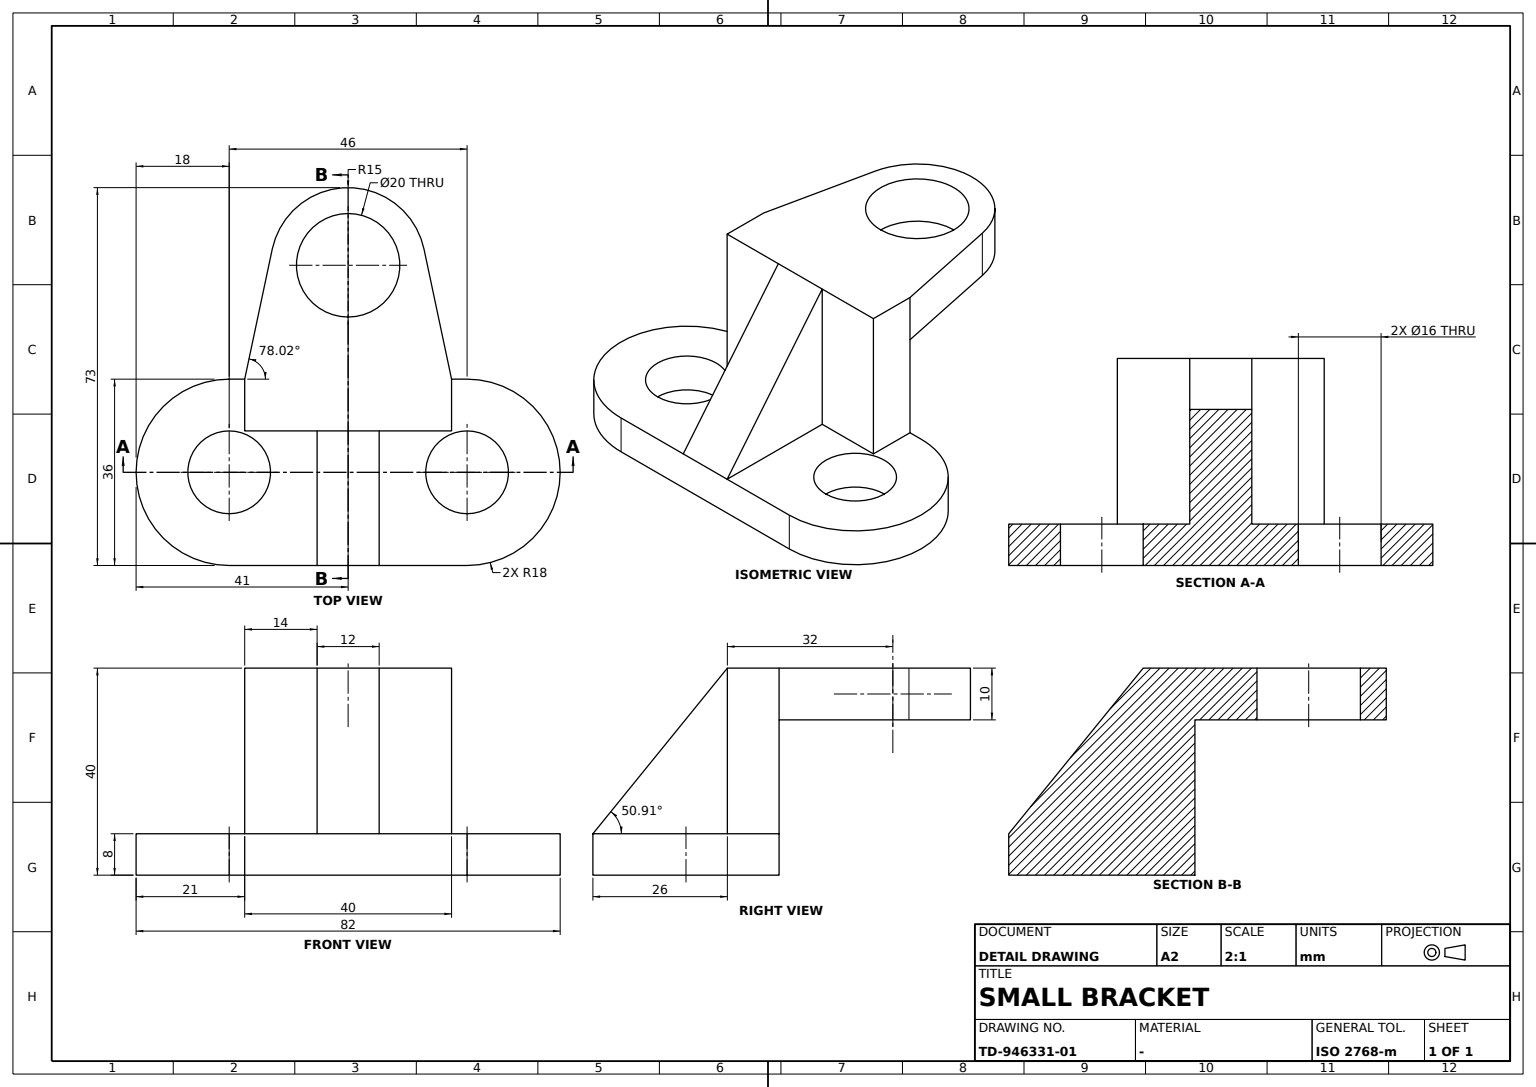
ISO-10303-21;
HEADER;
FILE_DESCRIPTION((''),'2;1');
FILE_NAME('','',(''),(''),'','','');
FILE_SCHEMA(('AUTOMOTIVE_DESIGN'));
ENDSEC;
DATA;
#1=APPLICATION_CONTEXT('');
#2=PRODUCT_CONTEXT('',#1,'mechanical');
#3=PRODUCT('','','',(#2));
#4=PRODUCT_DEFINITION_FORMATION('','',#3);
#5=PRODUCT_DEFINITION_CONTEXT('',#1,'design');
#6=PRODUCT_DEFINITION('','',#4,#5);
#7=PRODUCT_DEFINITION_SHAPE('','',#6);
#8=(LENGTH_UNIT()NAMED_UNIT(*)SI_UNIT(.MILLI.,.METRE.));
#9=(NAMED_UNIT(*)PLANE_ANGLE_UNIT()SI_UNIT($,.RADIAN.));
#10=(NAMED_UNIT(*)SI_UNIT($,.STERADIAN.)SOLID_ANGLE_UNIT());
#11=UNCERTAINTY_MEASURE_WITH_UNIT(LENGTH_MEASURE(0.005),#8,'distance_accuracy_value','');
#12=(GEOMETRIC_REPRESENTATION_CONTEXT(3)GLOBAL_UNCERTAINTY_ASSIGNED_CONTEXT((#11))GLOBAL_UNIT_ASSIGNED_CONTEXT((#8,#9,#10))REPRESENTATION_CONTEXT('',''));
#13=CARTESIAN_POINT('',(-30.,0.,26.));
#14=VERTEX_POINT('',#13);
#15=CARTESIAN_POINT('',(-40.,0.,26.));
#16=DIRECTION('',(0.,0.,1.));
#17=DIRECTION('',(1.,0.,0.));
#18=AXIS2_PLACEMENT_3D('',#15,#16,#17);
#19=CIRCLE('',#18,10.);
#20=EDGE_CURVE('',#14,#14,#19,.T.);
#21=ORIENTED_EDGE('',*,*,#20,.F.);
#22=EDGE_LOOP('',(#21));
#23=FACE_BOUND('',#22,.T.);
#24=CARTESIAN_POINT('',(-30.,0.,36.));
#25=VERTEX_POINT('',#24);
#26=CARTESIAN_POINT('',(-40.,0.,36.));
#27=AXIS2_PLACEMENT_3D('',#26,#16,#17);
#28=CIRCLE('',#27,10.);
#29=EDGE_CURVE('',#25,#25,#28,.T.);
#30=ORIENTED_EDGE('',*,*,#29,.T.);
#31=EDGE_LOOP('',(#30));
#32=FACE_BOUND('',#31,.T.);
#33=CARTESIAN_POINT('',(-40.,0.,31.));
#34=DIRECTION('',(0.,1.,0.));
#35=AXIS2_PLACEMENT_3D('',#33,#16,#34);
#36=CYLINDRICAL_SURFACE('',#35,10.);
#37=ADVANCED_FACE('',(#23,#32),#36,.F.);
#38=CARTESIAN_POINT('',(-8.,-20.,36.));
#39=VERTEX_POINT('',#38);
#40=CARTESIAN_POINT('',(-8.,-20.,4.));
#41=VERTEX_POINT('',#40);
#42=DIRECTION('',(0.,0.,-1.));
#43=VECTOR('',#42,1000.);
#44=LINE('',#38,#43);
#45=EDGE_CURVE('',#39,#41,#44,.T.);
#46=ORIENTED_EDGE('',*,*,#45,.T.);
#47=CARTESIAN_POINT('',(-8.,-6.,4.));
#48=VERTEX_POINT('',#47);
#49=CARTESIAN_POINT('',(-8.,0.,4.));
#50=DIRECTION('',(0.,-1.,0.));
#51=VECTOR('',#50,1000.);
#52=LINE('',#49,#51);
#53=EDGE_CURVE('',#48,#41,#52,.T.);
#54=ORIENTED_EDGE('',*,*,#53,.F.);
#55=CARTESIAN_POINT('',(-8.,-6.,36.));
#56=VERTEX_POINT('',#55);
#57=CARTESIAN_POINT('',(-8.,-6.,0.));
#58=LINE('',#57,#43);
#59=EDGE_CURVE('',#56,#48,#58,.T.);
#60=ORIENTED_EDGE('',*,*,#59,.F.);
#61=CARTESIAN_POINT('',(-8.,20.,36.));
#62=LINE('',#61,#51);
#63=EDGE_CURVE('',#56,#39,#62,.T.);
#64=ORIENTED_EDGE('',*,*,#63,.T.);
#65=EDGE_LOOP('',(#46,#54,#60,#64));
#66=FACE_BOUND('',#65,.T.);
#67=CARTESIAN_POINT('',(-8.,0.,0.));
#68=DIRECTION('',(-1.,0.,0.));
#69=AXIS2_PLACEMENT_3D('',#67,#68,#50);
#70=PLANE('',#69);
#71=ADVANCED_FACE('',(#66),#70,.F.);
#72=CARTESIAN_POINT('',(8.,23.,4.));
#73=VERTEX_POINT('',#72);
#74=CARTESIAN_POINT('',(0.,23.,4.));
#75=AXIS2_PLACEMENT_3D('',#74,#16,#17);
#76=CIRCLE('',#75,8.);
#77=EDGE_CURVE('',#73,#73,#76,.T.);
#78=ORIENTED_EDGE('',*,*,#77,.F.);
#79=EDGE_LOOP('',(#78));
#80=FACE_BOUND('',#79,.T.);
#81=CARTESIAN_POINT('',(-18.,20.,4.));
#82=VERTEX_POINT('',#81);
#83=CARTESIAN_POINT('',(-18.,23.,4.));
#84=VERTEX_POINT('',#83);
#85=CARTESIAN_POINT('',(-18.,0.,4.));
#86=VECTOR('',#34,1000.);
#87=LINE('',#85,#86);
#88=EDGE_CURVE('',#82,#84,#87,.T.);
#89=ORIENTED_EDGE('',*,*,#88,.F.);
#90=CARTESIAN_POINT('',(-8.,20.,4.));
#91=VERTEX_POINT('',#90);
#92=VECTOR('',#17,1000.);
#93=LINE('',#81,#92);
#94=EDGE_CURVE('',#82,#91,#93,.T.);
#95=ORIENTED_EDGE('',*,*,#94,.T.);
#96=CARTESIAN_POINT('',(-8.,6.,4.));
#97=VERTEX_POINT('',#96);
#98=EDGE_CURVE('',#91,#97,#52,.T.);
#99=ORIENTED_EDGE('',*,*,#98,.T.);
#100=CARTESIAN_POINT('',(18.,6.,4.));
#101=VERTEX_POINT('',#100);
#102=CARTESIAN_POINT('',(0.,6.,4.));
#103=LINE('',#102,#92);
#104=EDGE_CURVE('',#97,#101,#103,.T.);
#105=ORIENTED_EDGE('',*,*,#104,.T.);
#106=CARTESIAN_POINT('',(18.,23.,4.));
#107=VERTEX_POINT('',#106);
#108=CARTESIAN_POINT('',(18.,0.,4.));
#109=LINE('',#108,#51);
#110=EDGE_CURVE('',#107,#101,#109,.T.);
#111=ORIENTED_EDGE('',*,*,#110,.F.);
#112=CIRCLE('',#75,18.);
#113=EDGE_CURVE('',#107,#84,#112,.T.);
#114=ORIENTED_EDGE('',*,*,#113,.T.);
#115=EDGE_LOOP('',(#89,#95,#99,#105,#111,#114));
#116=FACE_BOUND('',#115,.T.);
#117=CARTESIAN_POINT('',(0.,0.,4.));
#118=AXIS2_PLACEMENT_3D('',#117,#16,#34);
#119=PLANE('',#118);
#120=ADVANCED_FACE('',(#80,#116),#119,.T.);
#121=CARTESIAN_POINT('',(-43.112329,14.673562,36.));
#122=VERTEX_POINT('',#121);
#123=CARTESIAN_POINT('',(-18.,20.,36.));
#124=VERTEX_POINT('',#123);
#125=DIRECTION('',(0.97823744,0.207488582,0.));
#126=VECTOR('',#125,1000.);
#127=LINE('',#121,#126);
#128=EDGE_CURVE('',#122,#124,#127,.T.);
#129=ORIENTED_EDGE('',*,*,#128,.T.);
#130=CARTESIAN_POINT('',(-18.,20.,26.));
#131=VERTEX_POINT('',#130);
#132=LINE('',#123,#43);
#133=EDGE_CURVE('',#124,#131,#132,.T.);
#134=ORIENTED_EDGE('',*,*,#133,.T.);
#135=CARTESIAN_POINT('',(-43.112329,14.673562,26.));
#136=VERTEX_POINT('',#135);
#137=LINE('',#135,#126);
#138=EDGE_CURVE('',#136,#131,#137,.T.);
#139=ORIENTED_EDGE('',*,*,#138,.F.);
#140=CARTESIAN_POINT('',(-43.112329,14.673562,31.));
#141=VECTOR('',#16,1000.);
#142=LINE('',#140,#141);
#143=EDGE_CURVE('',#122,#136,#142,.F.);
#144=ORIENTED_EDGE('',*,*,#143,.F.);
#145=EDGE_LOOP('',(#129,#134,#139,#144));
#146=FACE_BOUND('',#145,.T.);
#147=DIRECTION('',(-0.207488582,0.97823744,0.));
#148=AXIS2_PLACEMENT_3D('',#121,#147,#125);
#149=PLANE('',#148);
#150=ADVANCED_FACE('',(#146),#149,.T.);
#151=CARTESIAN_POINT('',(8.,23.,-4.));
#152=VERTEX_POINT('',#151);
#153=CARTESIAN_POINT('',(0.,23.,-4.));
#154=AXIS2_PLACEMENT_3D('',#153,#16,#17);
#155=CIRCLE('',#154,8.);
#156=EDGE_CURVE('',#152,#152,#155,.T.);
#157=ORIENTED_EDGE('',*,*,#156,.T.);
#158=EDGE_LOOP('',(#157));
#159=FACE_BOUND('',#158,.T.);
#160=CARTESIAN_POINT('',(8.,-23.,-4.));
#161=VERTEX_POINT('',#160);
#162=CARTESIAN_POINT('',(0.,-23.,-4.));
#163=AXIS2_PLACEMENT_3D('',#162,#16,#17);
#164=CIRCLE('',#163,8.);
#165=EDGE_CURVE('',#161,#161,#164,.T.);
#166=ORIENTED_EDGE('',*,*,#165,.T.);
#167=EDGE_LOOP('',(#166));
#168=FACE_BOUND('',#167,.T.);
#169=CARTESIAN_POINT('',(18.,23.,-4.));
#170=VERTEX_POINT('',#169);
#171=CARTESIAN_POINT('',(18.,-23.,-4.));
#172=VERTEX_POINT('',#171);
#173=CARTESIAN_POINT('',(18.,0.,-4.));
#174=LINE('',#173,#51);
#175=EDGE_CURVE('',#170,#172,#174,.T.);
#176=ORIENTED_EDGE('',*,*,#175,.T.);
#177=CARTESIAN_POINT('',(-18.,-23.,-4.));
#178=VERTEX_POINT('',#177);
#179=CIRCLE('',#163,18.);
#180=EDGE_CURVE('',#178,#172,#179,.T.);
#181=ORIENTED_EDGE('',*,*,#180,.F.);
#182=CARTESIAN_POINT('',(-18.,23.,-4.));
#183=VERTEX_POINT('',#182);
#184=CARTESIAN_POINT('',(-18.,0.,-4.));
#185=LINE('',#184,#86);
#186=EDGE_CURVE('',#178,#183,#185,.T.);
#187=ORIENTED_EDGE('',*,*,#186,.T.);
#188=CIRCLE('',#154,18.);
#189=EDGE_CURVE('',#170,#183,#188,.T.);
#190=ORIENTED_EDGE('',*,*,#189,.F.);
#191=EDGE_LOOP('',(#176,#181,#187,#190));
#192=FACE_BOUND('',#191,.T.);
#193=CARTESIAN_POINT('',(0.,0.,-4.));
#194=AXIS2_PLACEMENT_3D('',#193,#16,#34);
#195=PLANE('',#194);
#196=ADVANCED_FACE('',(#159,#168,#192),#195,.F.);
#197=ORIENTED_EDGE('',*,*,#20,.T.);
#198=EDGE_LOOP('',(#197));
#199=FACE_BOUND('',#198,.T.);
#200=ORIENTED_EDGE('',*,*,#138,.T.);
#201=CARTESIAN_POINT('',(-18.,-20.,26.));
#202=VERTEX_POINT('',#201);
#203=CARTESIAN_POINT('',(-18.,0.,26.));
#204=LINE('',#203,#86);
#205=EDGE_CURVE('',#202,#131,#204,.T.);
#206=ORIENTED_EDGE('',*,*,#205,.F.);
#207=CARTESIAN_POINT('',(-43.112329,-14.673562,26.));
#208=VERTEX_POINT('',#207);
#209=DIRECTION('',(-0.97823744,0.207488582,0.));
#210=VECTOR('',#209,1000.);
#211=LINE('',#201,#210);
#212=EDGE_CURVE('',#202,#208,#211,.T.);
#213=ORIENTED_EDGE('',*,*,#212,.T.);
#214=CIRCLE('',#18,15.);
#215=EDGE_CURVE('',#136,#208,#214,.T.);
#216=ORIENTED_EDGE('',*,*,#215,.F.);
#217=EDGE_LOOP('',(#200,#206,#213,#216));
#218=FACE_BOUND('',#217,.T.);
#219=CARTESIAN_POINT('',(0.,0.,26.));
#220=AXIS2_PLACEMENT_3D('',#219,#16,#34);
#221=PLANE('',#220);
#222=ADVANCED_FACE('',(#199,#218),#221,.F.);
#223=CARTESIAN_POINT('',(-18.,-20.,4.));
#224=VERTEX_POINT('',#223);
#225=CARTESIAN_POINT('',(-18.,-20.,0.));
#226=LINE('',#225,#43);
#227=EDGE_CURVE('',#202,#224,#226,.T.);
#228=ORIENTED_EDGE('',*,*,#227,.T.);
#229=CARTESIAN_POINT('',(0.,-20.,4.));
#230=LINE('',#229,#92);
#231=EDGE_CURVE('',#224,#41,#230,.T.);
#232=ORIENTED_EDGE('',*,*,#231,.T.);
#233=ORIENTED_EDGE('',*,*,#45,.F.);
#234=CARTESIAN_POINT('',(-18.,-20.,36.));
#235=VERTEX_POINT('',#234);
#236=LINE('',#234,#92);
#237=EDGE_CURVE('',#235,#39,#236,.T.);
#238=ORIENTED_EDGE('',*,*,#237,.F.);
#239=LINE('',#234,#43);
#240=EDGE_CURVE('',#235,#202,#239,.T.);
#241=ORIENTED_EDGE('',*,*,#240,.T.);
#242=EDGE_LOOP('',(#228,#232,#233,#238,#241));
#243=FACE_BOUND('',#242,.T.);
#244=AXIS2_PLACEMENT_3D('',#234,#50,#42);
#245=PLANE('',#244);
#246=ADVANCED_FACE('',(#243),#245,.T.);
#247=CARTESIAN_POINT('',(18.,23.,0.));
#248=LINE('',#247,#141);
#249=EDGE_CURVE('',#170,#107,#248,.T.);
#250=ORIENTED_EDGE('',*,*,#249,.F.);
#251=ORIENTED_EDGE('',*,*,#189,.T.);
#252=CARTESIAN_POINT('',(-18.,23.,0.));
#253=LINE('',#252,#141);
#254=EDGE_CURVE('',#183,#84,#253,.T.);
#255=ORIENTED_EDGE('',*,*,#254,.T.);
#256=ORIENTED_EDGE('',*,*,#113,.F.);
#257=EDGE_LOOP('',(#250,#251,#255,#256));
#258=FACE_BOUND('',#257,.T.);
#259=CARTESIAN_POINT('',(0.,23.,0.));
#260=AXIS2_PLACEMENT_3D('',#259,#16,#68);
#261=CYLINDRICAL_SURFACE('',#260,18.);
#262=ADVANCED_FACE('',(#258),#261,.T.);
#263=CARTESIAN_POINT('',(-8.,6.,36.));
#264=VERTEX_POINT('',#263);
#265=CARTESIAN_POINT('',(-8.,6.,0.));
#266=LINE('',#265,#43);
#267=EDGE_CURVE('',#264,#97,#266,.T.);
#268=ORIENTED_EDGE('',*,*,#267,.T.);
#269=ORIENTED_EDGE('',*,*,#98,.F.);
#270=VERTEX_POINT('',#61);
#271=LINE('',#90,#141);
#272=EDGE_CURVE('',#91,#270,#271,.T.);
#273=ORIENTED_EDGE('',*,*,#272,.T.);
#274=EDGE_CURVE('',#270,#264,#62,.T.);
#275=ORIENTED_EDGE('',*,*,#274,.T.);
#276=EDGE_LOOP('',(#268,#269,#273,#275));
#277=FACE_BOUND('',#276,.T.);
#278=ADVANCED_FACE('',(#277),#70,.F.);
#279=CARTESIAN_POINT('',(8.,-23.,4.));
#280=VERTEX_POINT('',#279);
#281=CARTESIAN_POINT('',(0.,-23.,4.));
#282=AXIS2_PLACEMENT_3D('',#281,#16,#17);
#283=CIRCLE('',#282,8.);
#284=EDGE_CURVE('',#280,#280,#283,.T.);
#285=ORIENTED_EDGE('',*,*,#284,.F.);
#286=EDGE_LOOP('',(#285));
#287=FACE_BOUND('',#286,.T.);
#288=ORIENTED_EDGE('',*,*,#231,.F.);
#289=CARTESIAN_POINT('',(-18.,-23.,4.));
#290=VERTEX_POINT('',#289);
#291=EDGE_CURVE('',#290,#224,#87,.T.);
#292=ORIENTED_EDGE('',*,*,#291,.F.);
#293=CARTESIAN_POINT('',(18.,-23.,4.));
#294=VERTEX_POINT('',#293);
#295=CIRCLE('',#282,18.);
#296=EDGE_CURVE('',#290,#294,#295,.T.);
#297=ORIENTED_EDGE('',*,*,#296,.T.);
#298=CARTESIAN_POINT('',(18.,-6.,4.));
#299=VERTEX_POINT('',#298);
#300=EDGE_CURVE('',#299,#294,#109,.T.);
#301=ORIENTED_EDGE('',*,*,#300,.F.);
#302=CARTESIAN_POINT('',(0.,-6.,4.));
#303=LINE('',#302,#92);
#304=EDGE_CURVE('',#48,#299,#303,.T.);
#305=ORIENTED_EDGE('',*,*,#304,.F.);
#306=ORIENTED_EDGE('',*,*,#53,.T.);
#307=EDGE_LOOP('',(#288,#292,#297,#301,#305,#306));
#308=FACE_BOUND('',#307,.T.);
#309=ADVANCED_FACE('',(#287,#308),#119,.T.);
#310=ORIENTED_EDGE('',*,*,#156,.F.);
#311=EDGE_LOOP('',(#310));
#312=FACE_BOUND('',#311,.T.);
#313=ORIENTED_EDGE('',*,*,#77,.T.);
#314=EDGE_LOOP('',(#313));
#315=FACE_BOUND('',#314,.T.);
#316=AXIS2_PLACEMENT_3D('',#259,#16,#34);
#317=CYLINDRICAL_SURFACE('',#316,8.);
#318=ADVANCED_FACE('',(#312,#315),#317,.F.);
#319=DIRECTION('',(-0.630592625,0.,0.776114));
#320=VECTOR('',#319,1000.);
#321=LINE('',#298,#320);
#322=EDGE_CURVE('',#299,#56,#321,.T.);
#323=ORIENTED_EDGE('',*,*,#322,.F.);
#324=EDGE_CURVE('',#101,#299,#109,.T.);
#325=ORIENTED_EDGE('',*,*,#324,.F.);
#326=LINE('',#100,#320);
#327=EDGE_CURVE('',#101,#264,#326,.T.);
#328=ORIENTED_EDGE('',*,*,#327,.T.);
#329=CARTESIAN_POINT('',(-8.,0.,36.));
#330=LINE('',#329,#51);
#331=EDGE_CURVE('',#264,#56,#330,.T.);
#332=ORIENTED_EDGE('',*,*,#331,.T.);
#333=EDGE_LOOP('',(#323,#325,#328,#332));
#334=FACE_BOUND('',#333,.T.);
#335=DIRECTION('',(0.776114,0.,0.630592625));
#336=DIRECTION('',(0.630592625,0.,-0.776114));
#337=AXIS2_PLACEMENT_3D('',#108,#335,#336);
#338=PLANE('',#337);
#339=ADVANCED_FACE('',(#334),#338,.T.);
#340=CARTESIAN_POINT('',(-43.112329,-14.673562,36.));
#341=VERTEX_POINT('',#340);
#342=CIRCLE('',#27,15.);
#343=EDGE_CURVE('',#122,#341,#342,.T.);
#344=ORIENTED_EDGE('',*,*,#343,.F.);
#345=ORIENTED_EDGE('',*,*,#143,.T.);
#346=ORIENTED_EDGE('',*,*,#215,.T.);
#347=CARTESIAN_POINT('',(-43.112329,-14.673562,31.));
#348=LINE('',#347,#141);
#349=EDGE_CURVE('',#341,#208,#348,.F.);
#350=ORIENTED_EDGE('',*,*,#349,.F.);
#351=EDGE_LOOP('',(#344,#345,#346,#350));
#352=FACE_BOUND('',#351,.T.);
#353=CYLINDRICAL_SURFACE('',#35,15.);
#354=ADVANCED_FACE('',(#352),#353,.T.);
#355=ORIENTED_EDGE('',*,*,#349,.T.);
#356=ORIENTED_EDGE('',*,*,#212,.F.);
#357=ORIENTED_EDGE('',*,*,#240,.F.);
#358=LINE('',#234,#210);
#359=EDGE_CURVE('',#235,#341,#358,.T.);
#360=ORIENTED_EDGE('',*,*,#359,.T.);
#361=EDGE_LOOP('',(#355,#356,#357,#360));
#362=FACE_BOUND('',#361,.T.);
#363=DIRECTION('',(-0.207488582,-0.97823744,0.));
#364=AXIS2_PLACEMENT_3D('',#234,#363,#209);
#365=PLANE('',#364);
#366=ADVANCED_FACE('',(#362),#365,.T.);
#367=ORIENTED_EDGE('',*,*,#267,.F.);
#368=ORIENTED_EDGE('',*,*,#327,.F.);
#369=ORIENTED_EDGE('',*,*,#104,.F.);
#370=EDGE_LOOP('',(#367,#368,#369));
#371=FACE_BOUND('',#370,.T.);
#372=CARTESIAN_POINT('',(0.,6.,0.));
#373=AXIS2_PLACEMENT_3D('',#372,#34,#68);
#374=PLANE('',#373);
#375=ADVANCED_FACE('',(#371),#374,.T.);
#376=ORIENTED_EDGE('',*,*,#284,.T.);
#377=EDGE_LOOP('',(#376));
#378=FACE_BOUND('',#377,.T.);
#379=ORIENTED_EDGE('',*,*,#165,.F.);
#380=EDGE_LOOP('',(#379));
#381=FACE_BOUND('',#380,.T.);
#382=CARTESIAN_POINT('',(0.,-23.,0.));
#383=AXIS2_PLACEMENT_3D('',#382,#16,#34);
#384=CYLINDRICAL_SURFACE('',#383,8.);
#385=ADVANCED_FACE('',(#378,#381),#384,.F.);
#386=ORIENTED_EDGE('',*,*,#300,.T.);
#387=CARTESIAN_POINT('',(18.,-23.,0.));
#388=LINE('',#387,#141);
#389=EDGE_CURVE('',#172,#294,#388,.T.);
#390=ORIENTED_EDGE('',*,*,#389,.F.);
#391=ORIENTED_EDGE('',*,*,#175,.F.);
#392=ORIENTED_EDGE('',*,*,#249,.T.);
#393=ORIENTED_EDGE('',*,*,#110,.T.);
#394=ORIENTED_EDGE('',*,*,#324,.T.);
#395=EDGE_LOOP('',(#386,#390,#391,#392,#393,#394));
#396=FACE_BOUND('',#395,.T.);
#397=CARTESIAN_POINT('',(18.,41.,0.));
#398=AXIS2_PLACEMENT_3D('',#397,#68,#50);
#399=PLANE('',#398);
#400=ADVANCED_FACE('',(#396),#399,.F.);
#401=ORIENTED_EDGE('',*,*,#29,.F.);
#402=EDGE_LOOP('',(#401));
#403=FACE_BOUND('',#402,.T.);
#404=ORIENTED_EDGE('',*,*,#274,.F.);
#405=LINE('',#123,#92);
#406=EDGE_CURVE('',#124,#270,#405,.T.);
#407=ORIENTED_EDGE('',*,*,#406,.F.);
#408=ORIENTED_EDGE('',*,*,#128,.F.);
#409=ORIENTED_EDGE('',*,*,#343,.T.);
#410=ORIENTED_EDGE('',*,*,#359,.F.);
#411=ORIENTED_EDGE('',*,*,#237,.T.);
#412=ORIENTED_EDGE('',*,*,#63,.F.);
#413=ORIENTED_EDGE('',*,*,#331,.F.);
#414=EDGE_LOOP('',(#404,#407,#408,#409,#410,#411,#412,#413));
#415=FACE_BOUND('',#414,.T.);
#416=AXIS2_PLACEMENT_3D('',#123,#16,#50);
#417=PLANE('',#416);
#418=ADVANCED_FACE('',(#403,#415),#417,.T.);
#419=ORIENTED_EDGE('',*,*,#254,.F.);
#420=ORIENTED_EDGE('',*,*,#186,.F.);
#421=CARTESIAN_POINT('',(-18.,-23.,0.));
#422=LINE('',#421,#141);
#423=EDGE_CURVE('',#178,#290,#422,.T.);
#424=ORIENTED_EDGE('',*,*,#423,.T.);
#425=ORIENTED_EDGE('',*,*,#291,.T.);
#426=ORIENTED_EDGE('',*,*,#227,.F.);
#427=ORIENTED_EDGE('',*,*,#205,.T.);
#428=CARTESIAN_POINT('',(-18.,20.,0.));
#429=LINE('',#428,#141);
#430=EDGE_CURVE('',#82,#131,#429,.T.);
#431=ORIENTED_EDGE('',*,*,#430,.F.);
#432=ORIENTED_EDGE('',*,*,#88,.T.);
#433=EDGE_LOOP('',(#419,#420,#424,#425,#426,#427,#431,#432));
#434=FACE_BOUND('',#433,.T.);
#435=CARTESIAN_POINT('',(-18.,-41.,0.));
#436=AXIS2_PLACEMENT_3D('',#435,#17,#34);
#437=PLANE('',#436);
#438=ADVANCED_FACE('',(#434),#437,.F.);
#439=ORIENTED_EDGE('',*,*,#272,.F.);
#440=ORIENTED_EDGE('',*,*,#94,.F.);
#441=ORIENTED_EDGE('',*,*,#430,.T.);
#442=ORIENTED_EDGE('',*,*,#133,.F.);
#443=ORIENTED_EDGE('',*,*,#406,.T.);
#444=EDGE_LOOP('',(#439,#440,#441,#442,#443));
#445=FACE_BOUND('',#444,.T.);
#446=AXIS2_PLACEMENT_3D('',#81,#34,#16);
#447=PLANE('',#446);
#448=ADVANCED_FACE('',(#445),#447,.T.);
#449=ORIENTED_EDGE('',*,*,#59,.T.);
#450=ORIENTED_EDGE('',*,*,#304,.T.);
#451=ORIENTED_EDGE('',*,*,#322,.T.);
#452=EDGE_LOOP('',(#449,#450,#451));
#453=FACE_BOUND('',#452,.T.);
#454=CARTESIAN_POINT('',(0.,-6.,0.));
#455=AXIS2_PLACEMENT_3D('',#454,#34,#68);
#456=PLANE('',#455);
#457=ADVANCED_FACE('',(#453),#456,.F.);
#458=ORIENTED_EDGE('',*,*,#296,.F.);
#459=ORIENTED_EDGE('',*,*,#423,.F.);
#460=ORIENTED_EDGE('',*,*,#180,.T.);
#461=ORIENTED_EDGE('',*,*,#389,.T.);
#462=EDGE_LOOP('',(#458,#459,#460,#461));
#463=FACE_BOUND('',#462,.T.);
#464=AXIS2_PLACEMENT_3D('',#382,#16,#50);
#465=CYLINDRICAL_SURFACE('',#464,18.);
#466=ADVANCED_FACE('',(#463),#465,.T.);
#467=CLOSED_SHELL('',(#37,#71,#120,#150,#196,#222,#246,#262,#278,#309,#318,#339,#354,#366,#375,#385,#400,#418,#438,#448,#457,#466));
#468=MANIFOLD_SOLID_BREP('',#467);
#469=ADVANCED_BREP_SHAPE_REPRESENTATION('',(#468),#12);
#470=SHAPE_DEFINITION_REPRESENTATION(#7,#469);
ENDSEC;
END-ISO-10303-21;
